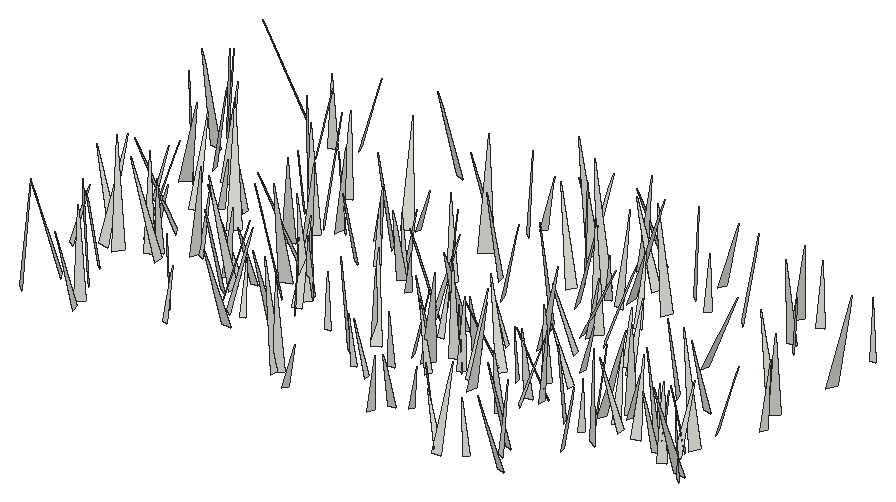
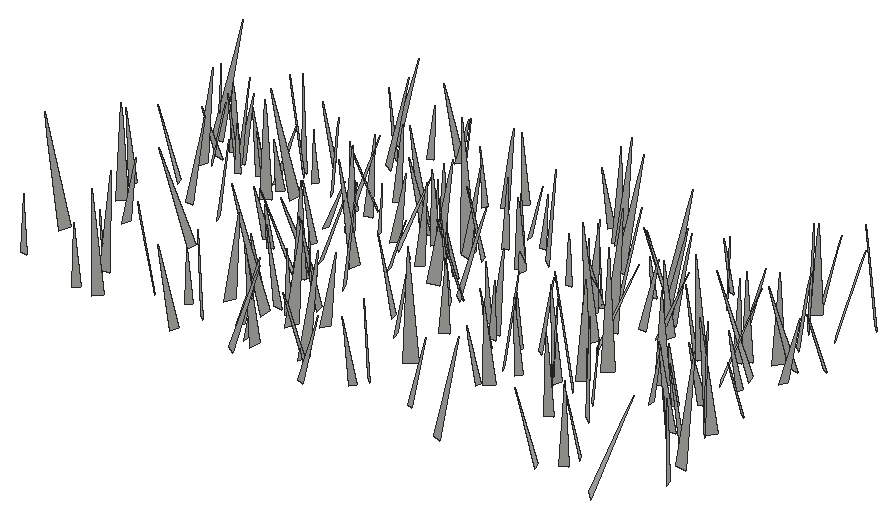
# SketchUp Ruby script. Lengths in inches.
U = 1.inch
M = Sketchup.active_model
def pt(a) = Geom::Point3d.new(a.map { |v| v * U })
def face(e, loops, mat)
  f = e.add_face(loops[0].map { |a| pt(a) })
  loops[1..].each { |l| e.add_face(l.map { |a| pt(a) }).erase! }
  f.material = f.back_material = mat if mat
  f
end
# faces: each face lists its corners as indices into pts; further lists are holes
def faces(e, pts, list, mat = nil) = list.each { |f| face(e, (f[0].is_a?(Array) ? f : [f]).map { |l| l.map { |i| pts[i] } }, mat) }
# xy, xz, yz: faces in a plane at the given z, y or x. An outline is a flat list of corners, or four numbers for a rectangle; further outlines are holes
def ring(l) = l.size == 4 ? [[l[0], l[1]], [l[2], l[1]], [l[2], l[3]], [l[0], l[3]]] : l.each_slice(2).to_a
def flat(e, list, mat, &to3) = list.each { |f| face(e, (f[0].is_a?(Array) ? f : [f]).map { |l| ring(l).map { |u, v| to3.(u, v) } }, mat) }
def xy(e, z, list, mat = nil) = flat(e, list, mat) { |x, y| [x, y, z] }
def xz(e, y, list, mat = nil) = flat(e, list, mat) { |x, z| [x, y, z] }
def yz(e, x, list, mat = nil) = flat(e, list, mat) { |y, z| [x, y, z] }
def lines(e, pts, list) = list.each { |a, b| e.add_line(pt(pts[a]), pt(pts[b])) }
# prism: a flat outline (further loops are holes) pulled along v
def prism(e, loops, v, mat = nil)
  f = face(e, loops, mat); d = Geom::Vector3d.new(v.map { |x| x * U })
  f.pushpull(f.normal.samedirection?(d) ? d.length : -d.length)
end
def box(e, o, s, mat = nil) = prism(e, [[o, [o[0] + s[0], o[1], o[2]], [o[0] + s[0], o[1] + s[1], o[2]], [o[0], o[1] + s[1], o[2]]]], [0, 0, s[2]], mat)
def at(x, y, z, deg = 0) = Geom::Transformation.translation(pt([x, y, z])) * Geom::Transformation.rotation(ORIGIN, Z_AXIS, deg.degrees)
def axes(o, x, y, z) = Geom::Transformation.new([*x, 0, *y, 0, *z, 0, *pt(o).to_a, 1])
def part(name) = M.definitions.add(name)
# library, detail: a bought-in or finely detailed component or shape, given as its bounding box
def library(name, o, s) = part(name).tap { |d| box(d.entities, o, s) }
def detail(e, o, s) = box(e.add_group.entities, o, s)
def put(e, d, t, mat = nil) = e.add_instance(d, t).tap { |i| i.material = mat if mat }
def group(e, t, mat = nil) = e.add_group.tap { |g| g.transformation = t; g.material = mat if mat }.entities
root = M.entities
c1 = part("fur_instance\#9")
p = [[0.8125,0,1.79],[0.67,-0.02,1.48],[0,-0.11,0],[0,0.11,0]]
faces(c1.entities,p,[[0,1,2,3]])
put(root,c1,axes([530.66,307.35,-21.66],[-1.81224,-5.34948,0.90018],[-5.42401,1.80193,-0.21131],[0.08596,0.92064,5.64415]))
put(root,c1,axes([467.42,306.52,-21.66],[-4.87581,-1.54153,0.97742],[-1.54685,4.96967,0.12147],[0.96896,0.17664,5.11224]))
put(root,c1,axes([498.44,307.21,-21.66],[3.31097,-1.72543,0.32906],[-1.73993,-3.31791,0.10944],[-0.24091,0.24944,3.73197]))
put(root,c1,axes([522.26,306.2,-21.66],[-3.36159,2.04077,0.19725],[2.04893,3.35754,0.1809],[0.07444,-0.25709,3.9284]))
put(root,c1,axes([459.37,306.45,-21.66],[4.78863,4.89843,2.46119],[5.13986,-5.14824,0.24599],[-1.90629,-1.57608,6.84581]))
put(root,c1,axes([522.34,305.76,-21.66],[-0.07417,5.83715,1.21265],[5.95855,0.11247,-0.17697],[0.19614,-1.2097,5.83493]))
put(root,c1,axes([525.3125,307.57,-21.66],[-2.21806,2.84038,1.31516],[3.07662,2.27502,0.2754],[0.57601,-1.21396,3.59328]))
put(root,c1,axes([509.79,309.11,-21.66],[3.72524,-2.31212,0.81738],[-2.32656,-3.80205,-0.15146],[-0.77532,0.29988,4.38182]))
put(root,c1,axes([466.73,308.3125,-21.66],[3.45962,-4.50001,2.91683],[-5.02174,-3.93643,-0.1168],[-1.88153,2.2319,5.67498]))
put(root,c1,axes([495.38,309.34,-21.66],[-7.11208,1.53537,2.26223],[1.65379,7.4363,0.15223],[2.17716,-0.6331,7.27433]))
put(root,c1,axes([495.52,309.58,-21.66],[3.10657,-5.20372,2.6425],[-5.63717,-3.45056,-0.16782],[-1.51121,2.17421,6.05816]))
put(root,c1,axes([511.11,311.35,-21.66],[1.53045,-4.60076,0.23907],[-4.60681,-1.52625,0.11946],[0.03806,0.26453,4.84716]))
put(root,c1,axes([518.17,310.44,-21.66],[-3.06281,-3.15709,1.43812],[-3.29391,3.24851,0.11628],[1.08883,0.94666,4.3971]))
put(root,c1,axes([528.46,310.15,-21.66],[-2.24155,-3.80564,2.54295],[-4.42537,2.52493,-0.12217],[1.16862,2.26183,4.41503]))
put(root,c1,axes([461.24,311.66,-21.66],[-5.49942,-3.45806,0.94275],[-3.51329,5.5426,-0.16378],[0.70973,0.64178,6.49422]))
put(root,c1,axes([477.7,310.56,-21.66],[1.06055,3.50039,1.15885],[3.68372,-1.05849,-0.17402],[-0.16095,-1.16074,3.65339]))
put(root,c1,axes([527.93,312.2,-21.66],[-2.71876,-5.31687,1.33657],[-5.469,2.73415,-0.24823],[0.3815,1.3048,5.9665]))
put(root,c1,axes([464.92,312.15,-21.66],[4.55418,4.59674,3.34406],[5.23121,-5.06575,-0.16086],[-2.22422,-2.50228,6.46875]))
put(root,c1,axes([513.14,312.56,-21.66],[3.09975,-1.98369,0.33098],[-1.98147,-3.11644,-0.1208],[-0.34401,0.07615,3.67817]))
put(root,c1,axes([483.9,314.35,-21.66],[0.0355,-6.28923,0.69696],[-6.32457,-0.05728,-0.19472],[-0.19984,0.69551,6.28631]))
put(root,c1,axes([491.09,314.8,-21.66],[-1.0754,-7.3325,1.08617],[-7.40599,1.10888,0.15329],[0.31086,1.05196,7.40935]))
put(root,c1,axes([475.96,313.58,-21.66],[3.3067,2.95122,2.18217],[3.23124,-3.73382,0.15332],[-1.74087,-1.32466,4.4295]))
put(root,c1,axes([504.39,315.08,-21.66],[-3.7389,-0.44853,0.79303],[-0.43438,3.82202,0.11371],[0.80087,-0.02096,3.764]))
put(root,c1,axes([463.32,316.11,-21.66],[-2.97615,-4.05495,1.48787],[-4.26463,3.04523,-0.23114],[0.68511,1.34083,5.02461]))
put(root,c1,axes([501.67,316.05,-21.66],[0.6335,-3.36408,1.34348],[-3.58683,-0.77327,-0.24494],[-0.50657,1.2682,3.41444]))
put(root,c1,axes([533.28,315.68,-21.66],[4.00682,1.30969,1.18737],[1.29487,-4.17692,0.23764],[-1.20352,-0.13365,4.20874]))
put(root,c1,axes([547.74,319.59,-21.66],[-0.40558,-7.48594,0.6627],[-7.51279,0.42075,0.15485],[0.19107,0.65318,7.49532]))
put(root,c1,axes([521.9,318.14,-21.66],[2.34766,-4.1804,1.05082],[-4.25289,-2.44131,-0.21062],[-0.70205,0.80976,4.78987]))
put(root,c1,axes([505.07,318.8125,-21.66],[1.42662,-4.11071,0.89066],[-4.20545,-1.41051,0.22612],[-0.07357,0.91596,4.34535]))
put(root,c1,axes([484.17,317.05,-21.66],[-1.12302,3.48075,0.37457],[3.50037,1.10997,0.18007],[-0.0574,-0.41163,3.65299]))
put(root,c1,axes([498.94,318.61,-21.66],[3.12486,4.78234,3.10342],[5.39282,-3.6275,0.15986],[-1.8492,-2.49745,5.71052]))
put(root,c1,axes([482,317.03,-21.66],[3.27247,4.57721,0.86039],[4.6176,-3.3258,0.13012],[-0.60735,-0.62316,5.62521]))
put(root,c1,axes([548.35,318.53,-21.66],[-3.07714,-3.38347,1.94932],[-3.73457,3.27489,-0.21099],[1.14047,1.59489,4.5686]))
put(root,c1,axes([535.08,319.03,-21.66],[-2.81459,-5.30869,2.75415],[-5.79641,3.17103,0.18862],[1.47279,2.33491,6.00571]))
put(root,c1,axes([457.4375,318.29,-21.66],[2.29816,3.3477,0.63042],[3.39972,-2.30202,-0.16916],[-0.21536,-0.61617,4.05709]))
put(root,c1,axes([478.39,320.55,-21.66],[-3.05463,-4.97038,1.37571],[-5.09206,3.16016,0.11108],[0.81742,1.11209,5.83293]))
put(root,c1,axes([479.4375,319.34,-21.66],[5.1332,2.66859,0.80867],[2.72409,-5.16107,-0.26035],[-0.59552,-0.60587,5.77956]))
put(root,c1,axes([534.64,319.73,-21.66],[5.13574,3.88277,2.0176],[4.11622,-5.34233,-0.19668],[-1.48436,-1.3806,6.4353]))
put(root,c1,axes([515.94,320.37,-21.66],[6.14943,-1.42717,1.61929],[-1.52874,-6.3314,0.22535],[-1.52376,0.59247,6.30885]))
put(root,c1,axes([507.93,322.17,-21.66],[6.18232,-5.30847,0.7026],[-5.32058,-6.21081,-0.10875],[-0.60412,0.37485,8.14795]))
put(root,c1,axes([532.21,320.52,-21.66],[-2.65217,1.9255,1.58872],[2.09556,2.97695,-0.10973],[1.35655,-0.83418,3.2756]))
put(root,c1,axes([509.6,320.11,-21.66],[-4.39525,1.44739,0.73649],[1.42922,4.45652,-0.22883],[0.77116,-0.01,4.62177]))
put(root,c1,axes([529.07,321.37,-21.66],[4.09073,2.15745,2.5023],[2.51133,-4.61824,-0.12369],[-2.14694,-1.2913,4.62314]))
put(root,c1,axes([544.28,320.54,-21.66],[-3.13208,3.88614,1.48189],[4.03166,3.29255,-0.11327],[1.02167,-1.07935,4.98991]))
put(root,c1,axes([542.07,322.125,-21.66],[0.17037,-4.40384,1.04145],[-4.5148,-0.2364,-0.26107],[-0.30825,1.02847,4.3994]))
put(root,c1,axes([493.76,321.06,-21.66],[-0.42673,3.51272,1.26133],[3.73148,0.37463,0.21911],[-0.0791,-1.27778,3.53176]))
put(root,c1,axes([467.84,321.62,-21.66],[-6.68615,-0.01766,0.93467],[0.01232,6.74773,0.2156],[0.93476,-0.21523,6.6827]))
put(root,c1,axes([462.76,320.43,-21.66],[-5.4488,4.52209,1.619],[4.59694,5.6194,-0.22458],[1.39234,-0.85616,7.07731]))
put(root,c1,axes([479.05,321.7,-21.66],[-7.32255,-0.11088,1.35528],[-0.08815,7.44603,0.13288],[1.35695,-0.11461,7.32218]))
put(root,c1,axes([488.25,321.68,-21.66],[-3.74017,-2.83655,2.38458],[-3.12746,4.23356,0.13062],[1.98777,1.32365,4.69232]))
put(root,c1,axes([499.97,321.9375,-21.66],[-4.58199,0.67037,2.42399],[0.81188,5.16228,0.10702],[2.38033,-0.47034,4.62953]))
put(root,c1,axes([522.46,322.8125,-21.66],[1.7038,-4.78318,1.39426],[-4.94528,-1.80274,-0.14134],[-0.60574,1.26373,5.0756]))
put(root,c1,axes([543.2,321.7,-21.66],[3.76786,2.01641,1.4087],[2.07515,-3.9894,0.15999],[-1.32064,-0.51569,4.27049]))
put(root,c1,axes([522.62,320.92,-21.66],[3.07177,3.42083,0.35758],[3.42072,-3.08846,0.16062],[-0.35863,-0.15826,4.59478]))
put(root,c1,axes([507.41,323.25,-21.66],[-0.73911,-5.79285,1.55471],[-5.99778,0.70592,-0.22109],[-0.03032,1.57006,5.83563]))
put(root,c1,axes([466.78,323.17,-21.66],[0.54293,-5.17192,1.62827],[-5.42158,-0.49338,0.24063],[0.08095,1.64396,5.19477]))
put(root,c1,axes([460.59,320.35,-21.66],[0.90222,6.95991,0.72818],[6.98982,-0.93156,0.24337],[-0.33621,-0.69025,7.01392]))
put(root,c1,axes([524.17,324.27,-21.66],[-3.22391,-4.50813,0.36238],[-4.51102,3.23719,0.13952],[0.32445,0.21334,5.54053]))
put(root,c1,axes([505.49,322.5,-21.66],[4.51759,1.55237,1.02195],[1.60919,-4.61101,-0.10928],[-0.92991,-0.4377,4.77562]))
put(root,c1,axes([480.32,324.07,-21.66],[-0.08561,-4.51883,0.61864],[-4.55746,0.06047,-0.18896],[-0.17898,0.62161,4.51569]))
put(root,c1,axes([466.05,322.18,-21.66],[-2.20554,5.93145,2.00046],[6.2413,2.24627,0.22087],[0.47966,-1.95462,6.32437]))
put(root,c1,axes([500.67,321.5625,-21.66],[-3.10471,5.12305,0.88051],[5.18598,3.12286,0.11631],[0.35573,-0.81381,5.98927]))
put(root,c1,axes([484.55,323.83,-21.66],[-5.73221,-5.07274,1.73381],[-5.23258,5.8463,-0.19467],[1.1657,1.29813,7.652]))
put(root,c1,axes([512.32,322.89,-21.66],[2.78644,2.89477,1.9564],[3.12581,-3.18339,0.25829],[-1.56092,-1.20736,4.00964]))
put(root,c1,axes([541.58,323.13,-21.66],[-6.14594,-1.15799,1.95321],[-1.28361,6.42082,-0.2323],[1.87305,0.60056,6.24977]))
put(root,c1,axes([514.49,321.92,-21.66],[0.1573,5.82785,1.1486],[5.93788,-0.12389,-0.18455],[0.15705,-1.15268,5.82705]))
put(root,c1,axes([512.07,323.25,-21.66],[-2.98009,3.50221,2.17702],[3.82104,3.35523,-0.16707],[1.55067,-1.53712,4.59549]))
put(root,c1,axes([476.6,323.46,-21.66],[4.38951,-2.01268,1.547],[-2.15257,-4.58905,0.13732],[-1.34555,0.7756,4.82698]))
put(root,c1,axes([524.23,323.125,-21.66],[4.53301,0.32886,1.81446],[0.26511,-4.88148,0.22244],[-1.82486,0.10775,4.53948]))
put(root,c1,axes([535.8,323.46,-21.66],[-4.77809,0.40303,0.49366],[0.4272,4.79644,0.21897],[0.47289,-0.2608,4.79006]))
put(root,c1,axes([544.7,324.4,-21.66],[-3.48684,-2.54111,1.02639],[-2.66037,3.53733,-0.28017],[0.65812,0.83597,4.30544]))
put(root,c1,axes([459.46,323.64,-21.66],[-4.99004,2.24313,0.58277],[2.2784,5.00139,0.2583],[0.42444,-0.4756,5.46492]))
put(root,c1,axes([538.38,323.07,-21.66],[-2.22109,4.73282,1.14399],[4.81333,2.32397,-0.26934],[0.73496,-0.91711,5.22114]))
put(root,c1,axes([477.6875,324.09,-21.66],[-5.92651,0.06077,0.05927],[0.05827,5.92175,-0.24529],[0.06173,0.24468,5.92174]))
put(root,c1,axes([544.89,322.75,-21.66],[0.14678,4.73777,0.12743],[4.7339,-0.15274,0.22615],[-0.23006,-0.12022,4.73465]))
put(root,c1,axes([531.96,324.78,-21.66],[6.74375,-1.56753,0.95704],[-1.61805,-6.79399,0.27364],[-0.86892,0.48558,6.91813]))
put(root,c1,axes([470.56,325.22,-21.66],[5.91489,-2.56905,1.81184],[-2.61095,-6.16477,-0.21752],[-1.75092,0.51416,6.44505]))
put(root,c1,axes([540.88,324.26,-21.66],[-1.02276,3.4571,1.0392],[3.60758,1.01767,0.16502],[0.12981,-1.04418,3.60144]))
put(root,c1,axes([487.22,325.95,-21.66],[2.10827,-4.41232,0.88185],[-4.4927,-2.11805,0.1432],[-0.24874,0.85808,4.88803]))
put(root,c1,axes([509.66,324.89,-21.66],[-1.05184,5.80364,2.59591],[6.34975,1.09094,0.13387],[0.3189,-2.57972,5.89666]))
put(root,c1,axes([487.54,324.6,-21.66],[-5.4066,3.91291,1.98693],[4.14231,5.59139,0.26032],[1.44915,-1.38406,6.66892]))
put(root,c1,axes([487.61,322.93,-21.66],[-1.13883,5.42731,0.08742],[5.42427,1.13458,0.2244],[-0.2017,-0.13157,5.54096]))
put(root,c1,axes([482.97,326.68,-21.66],[2.46891,-7.20313,1.70316],[-7.36136,-2.57683,-0.22704],[-0.77207,1.53499,7.61111]))
put(root,c1,axes([514.81,326.84,-21.66],[-3.4454,-3.89131,0.03074],[-3.88746,3.44363,0.20759],[0.17579,-0.11462,5.19326]))
put(root,c1,axes([518.83,325.27,-21.66],[3.01328,1.01562,1.71575],[1.06477,-3.44849,0.1713],[-1.68569,-0.36275,3.17522]))
put(root,c1,axes([471.23,325.33,-21.66],[1.95636,4.4496,1.57567],[4.70552,-1.97342,-0.26957],[-0.3738,-1.55425,4.8532]))
put(root,c1,axes([487.67,325.6,-21.66],[2.36348,3.65871,1.87372],[3.9267,-2.64879,0.21906],[-1.21573,-1.4425,4.3502]))
put(root,c1,axes([534.76,326.47,-21.66],[3.71508,-1.29272,0.27873],[-1.28155,-3.72443,-0.19222],[-0.32626,-0.0905,3.92887]))
put(root,c1,axes([462.98,325.3,-21.66],[6.72571,2.73267,0.89443],[2.78268,-6.75899,-0.27437],[-0.72399,-0.59256,7.25447]))
put(root,c1,axes([534.37,324.48,-21.66],[-2.34195,3.99616,0.3444],[3.99913,2.35703,-0.15486],[0.30802,-0.21845,4.62925]))
put(root,c1,axes([545.4,325.4,-21.66],[-6.9298,2.98954,1.57704],[3.02348,7.09089,-0.15622],[1.51094,-0.47802,7.54553]))
put(root,c1,axes([521.89,326.9375,-21.66],[4.08918,-3.36848,1.98263],[-3.52303,-4.41912,-0.24183],[-1.69286,1.05996,5.29241]))
put(root,c1,axes([510.38,328.24,-21.66],[2.722,-4.21365,0.18087],[-4.20663,-2.72794,-0.24377],[-0.30292,0.01939,5.01046]))
put(root,c1,axes([465.27,328.2,-21.66],[-5.5722,-4.07145,0.43281],[-4.071,5.58734,0.1482],[0.43699,0.13539,6.89957]))
put(root,c1,axes([516.1,325.6875,-21.66],[-4.785,3.6619,0.62252],[3.69492,4.79647,0.18627],[0.38032,-0.52686,6.02254]))
put(root,c1,axes([534.39,327.08,-21.66],[-1.98157,5.41612,3.08152],[6.10168,2.34277,-0.19399],[1.26474,-2.81671,5.76397]))
put(root,c1,axes([462.39,328.2,-21.66],[3.14021,-1.95272,0.11029],[-1.95573,-3.13292,0.21476],[0.01996,0.24059,3.6916]))
put(root,c1,axes([506.39,330.7,-21.66],[2.6634,-7.09113,0.13913],[-7.08626,-2.66678,-0.26525],[-0.29724,0.03689,7.57017]))
put(root,c1,axes([524.63,328.01,-21.66],[-3.98782,0.86871,0.11292],[0.87287,3.98492,0.16912],[0.07423,-0.18933,4.07783]))
put(root,c1,axes([505.36,327.8,-21.66],[0.0321,3.78164,0.61426],[3.82721,-0.05969,0.16749],[-0.17489,-0.6122,3.77806]))
put(root,c1,axes([483.15,329.96,-21.66],[6.93717,-2.75986,2.51351],[-2.97128,-7.29338,0.19237],[-2.25967,1.11744,7.46352]))
put(root,c1,axes([481.44,331.18,-21.66],[-5.39414,-3.77764,0.22745],[-3.78403,5.38986,-0.22257],[0.05845,0.31282,6.58162]))
put(root,c1,axes([501.96,331.6,-21.66],[-3.86878,-4.9807,0.99535],[-5.05831,3.89149,-0.18804],[0.45997,0.9025,6.30392]))
put(root,c1,axes([544.89,330.22,-21.66],[4.65489,2.00226,0.76997],[2.06003,-4.68544,-0.26978],[-0.59848,-0.55448,5.06006]))
put(root,c1,axes([512.64,331.13,-21.66],[-3.89073,-0.42692,0.42553],[-0.44504,3.90915,-0.14719],[0.40654,0.19356,3.91132]))
put(root,c1,axes([523.32,331.94,-21.66],[3.83276,-0.80553,0.30542],[-0.78769,-3.84079,-0.24507],[-0.34886,-0.17786,3.90882]))
put(root,c1,axes([540.79,333.45,-21.66],[-1.08369,-5.40972,1.03151],[-5.49173,1.14023,0.21038],[0.41232,0.96864,5.51318]))
put(root,c1,axes([501.6,331.24,-21.66],[3.62165,4.35293,0.90177],[4.41878,-3.65214,-0.11732],[-0.48531,-0.76904,5.66132]))
put(root,c1,axes([477.28,334.29,-21.66],[4.02071,-6.30995,0.86141],[-6.36147,-4.02715,0.19326],[-0.29869,0.83076,7.47959]))
put(root,c1,axes([516.22,333.16,-21.66],[6.40795,-1.734,1.03011],[-1.73088,-6.48917,-0.15614],[-1.03535,0.11648,6.63658]))
put(root,c1,axes([495.57,333.9375,-21.66],[2.79472,-2.37927,0.19168],[-2.37504,-2.80125,-0.14262],[-0.23842,0.01542,3.66757]))
put(root,c1,axes([458.3,332.66,-21.66],[2.21445,2.95218,0.72503],[3.03203,-2.20951,-0.26401],[-0.21871,-0.73996,3.68096]))
put(root,c1,axes([501.79,333.32,-21.66],[5.69134,3.55142,2.30083],[3.82093,-5.97012,-0.23634],[-1.81848,-1.42926,6.70433]))
put(root,c1,axes([535.89,334.13,-21.66],[4.40996,1.53054,2.75088],[1.88618,-5.07543,-0.19988],[-2.52036,-1.1203,4.66373]))
put(root,c1,axes([548.86,334.06,-21.66],[4.44334,-1.86269,1.64457],[-2.02269,-4.66849,0.17731],[-1.44323,0.80817,4.81471]))
put(root,c1,axes([520.02,334.68,-21.66],[-4.58656,-0.99691,0.53395],[-0.9871,4.61746,0.14195],[0.55187,-0.02624,4.69151]))
put(root,c1,axes([493.13,335.72,-21.66],[2.16413,-4.87719,1.14426],[-4.95965,-2.26151,-0.2591],[-0.70577,0.93721,5.32947]))
put(root,c1,axes([470.29,332.83,-21.66],[-5.1988,6.07272,1.14347],[6.1224,5.26442,-0.12263],[0.83765,-0.78798,7.99315]))
put(root,c1,axes([486.35,335.67,-21.66],[-2.7828,-3.97435,1.2381],[-4.07565,2.90431,0.16237],[0.84701,0.91751,4.84903]))
put(root,c1,axes([465.95,335.78,-21.66],[3.13443,-2.25979,0.73802],[-2.32723,-3.16608,0.18952],[-0.4851,0.5876,3.85946]))
put(root,c1,axes([463.53,333.66,-21.66],[-2.14385,5.53708,0.23418],[5.53457,2.15208,-0.21752],[0.2875,-0.13964,5.93364]))
put(root,c1,axes([528.35,334.49,-21.66],[-1.52341,4.48001,0.30788],[4.47725,1.54034,-0.26007],[0.34571,-0.20714,4.72479]))
put(root,c1,axes([492.76,336.62,-21.66],[-0.42877,3.87256,1.55947],[4.17346,0.35848,0.25729],[-0.1042,-1.57711,3.88772]))
put(root,c1,axes([526.67,335.92,-21.66],[-1.83169,3.1238,0.57494],[3.14275,1.87858,-0.19441],[0.4602,-0.39568,3.61599]))
put(root,c1,axes([468.62,336.93,-21.66],[-3.8802,0.07929,1.10053],[0.11582,4.03064,0.11798],[1.09728,-0.14508,3.87922]))
put(root,c1,axes([488.75,336.62,-21.66],[-3.06481,2.41196,1.362],[2.48233,3.29293,-0.24563],[1.22908,-0.63618,3.89234]))
put(root,c1,axes([458.44,338.36,-21.66],[5.57249,-4.36069,0.56036],[-4.38496,-5.5781,0.19774],[-0.31889,0.50141,7.07313]))
put(root,c1,axes([547.42,337.86,-21.66],[-3.8078,3.44308,3.43375],[4.19662,4.52997,0.11149],[2.45637,-2.40193,5.13242]))
put(root,c1,axes([513.98,337.91,-21.66],[-6.04607,-3.24149,2.31572],[-3.3744,6.40425,0.15438],[2.11738,0.95032,6.85845]))
put(root,c1,axes([478.23,337.77,-21.66],[-4.52139,5.22079,2.42729],[5.56937,4.74843,0.161],[1.45961,-1.94607,6.90462]))
put(root,c1,axes([459.07,339,-21.66],[-4.9247,-5.05159,2.9073],[-5.39927,5.38751,0.21521],[2.19519,1.91829,7.05159]))
put(root,c1,axes([518.82,338.69,-21.66],[4.01363,-0.60213,1.19124],[-0.70216,-4.16285,0.26162],[-1.13516,0.446,4.0501]))
put(root,c1,axes([491.41,338.9,-21.66],[3.83893,-0.81047,1.08867],[-0.8917,-3.9684,0.19003],[-1.0232,0.41758,3.91895]))
put(root,c1,axes([518.03,338.52,-21.66],[5.44846,0.74036,0.07595],[0.73692,-5.44519,0.21553],[-0.10422,0.20337,5.4943]))
put(root,c1,axes([521.3,338.55,-21.66],[4.74716,3.3592,0.52437],[3.38285,-4.75689,-0.1518],[-0.33985,-0.42721,5.81349]))
put(root,c1,axes([480.22,340.1,-21.66],[5.9168,-1.45412,1.7202],[-1.44139,-6.15974,-0.24915],[-1.73089,0.15879,6.08776]))
put(root,c1,axes([498.02,339.09,-21.66],[2.13883,-4.28297,3.06723],[-5.00629,-2.68295,-0.2554],[-1.63976,2.60467,4.7805]))
put(root,c1,axes([505.16,339.63,-21.66],[5.01565,1.80166,1.23073],[1.89818,-5.12441,-0.23415],[-1.07592,-0.64182,5.32428]))
put(root,c1,axes([480.64,340.59,-21.66],[-3.25997,-4.21096,1.97124],[-4.4396,3.53441,0.20814],[1.38129,1.42168,5.3213]))
put(root,c1,axes([484.92,341.45,-21.66],[3.8804,-2.67072,0.47699],[-2.66948,-3.90717,-0.15997],[-0.48385,0.13783,4.70793]))
put(root,c1,axes([487.4,341.15,-21.66],[-5.57513,-2.9786,1.92177],[-3.03694,5.86084,0.2736],[1.82819,0.65252,6.315]))
put(root,c1,axes([519.27,339.77,-21.66],[-5.69,4.35692,2.08043],[4.49689,5.95288,-0.16772],[1.75752,-1.1258,7.16454]))
put(root,c1,axes([477.97,340.07,-21.66],[5.88152,4.86813,2.28116],[5.13014,-6.09312,-0.22398],[-1.60749,-1.63397,7.63157]))
put(root,c1,axes([473.96,341.39,-21.66],[-3.08736,-2.6391,1.38175],[-2.74426,3.29386,0.15946],[1.15895,0.7691,4.05847]))
put(root,c1,axes([534.06,341.42,-21.66],[6.32443,-0.86949,0.03215],[-0.87008,-6.31952,0.24926],[0.00213,0.25131,6.37905]))
put(root,c1,axes([474.44,341.64,-21.66],[2.40837,2.51325,1.53163],[2.71206,-2.66382,0.10655],[-1.14326,-1.0248,3.47927]))
put(root,c1,axes([462.55,340.93,-21.66],[-0.45657,6.34549,1.8425],[6.59681,0.54314,-0.23589],[0.37708,-1.81886,6.35752]))
put(root,c1,axes([543.77,341.6,-21.66],[-4.87029,1.64927,0.93909],[1.65484,4.95663,-0.12272],[0.92923,-0.18296,5.1405]))
put(root,c1,axes([502.15,343.06,-21.66],[-5.31437,-1.63311,1.48269],[-1.72892,5.48589,-0.1545],[1.36976,0.58821,5.55749]))
put(root,c1,axes([459.34,342.84,-21.66],[5.12051,1.66894,1.66295],[1.70709,-5.37015,0.13306],[-1.62376,-0.38277,5.38398]))
put(root,c1,axes([513.03,343.8,-21.66],[5.83146,1.27805,1.15338],[1.33487,-5.92923,-0.17895],[-1.08712,-0.42484,5.96719]))
put(root,c1,axes([472.03,344.78,-21.66],[3.78368,4.97369,3.03573],[5.56614,-4.15585,-0.12867],[-1.72376,-2.50217,6.24798]))
put(root,c1,axes([522,343.89,-21.66],[-1.31854,4.49628,0.43937],[4.51767,1.31381,0.11263],[0.01505,-0.45333,4.68427]))
put(root,c1,axes([456.17,346.95,-21.66],[-0.95753,-7.17721,1.84222],[-7.39469,1.0444,0.22542],[0.47406,1.79439,7.23729]))
put(root,c1,axes([487.26,346.18,-21.66],[3.61055,-0.61097,0.20103],[-0.59508,-3.6081,-0.27795],[-0.24409,-0.24103,3.65131]))
put(root,c1,axes([515.02,347.13,-21.66],[2.03296,-3.43324,0.36978],[-3.45285,-2.01606,0.26469],[0.04074,0.45292,3.9812]))
put(root,c1,axes([548.43,347.26,-21.66],[6.87118,-2.4682,1.14103],[-2.53265,-6.93781,0.24398],[-0.98977,0.61792,7.29696]))
put(root,c1,axes([486.15,345.46,-21.66],[-3.98192,5.65644,1.02142],[5.69703,4.04883,-0.21229],[0.76316,-0.7113,6.91418]))
put(root,c1,axes([476.07,346.9,-21.66],[-2.39493,4.93051,2.15105],[5.27679,2.61079,-0.10925],[1.04521,-1.88321,5.4803]))
put(root,c1,axes([496.72,347,-21.66],[4.92232,-5.34816,3.43981],[-5.97476,-5.37881,0.1869],[-2.17654,2.67018,7.26616]))
put(root,c1,axes([517.0625,346.49,-21.66],[1.06492,5.99669,1.55027],[6.17359,-1.15473,0.22589],[-0.50038,-1.48458,6.08632]))
put(root,c1,axes([509.93,346.51,-21.66],[-5.57386,3.34507,0.61319],[3.34749,5.6042,-0.14346],[0.5998,-0.19191,6.49898]))
put(root,c1,axes([517.41,348.4375,-21.66],[8.28106,0.30024,0.90595],[0.31898,-8.32832,-0.15571],[-0.89952,-0.18935,8.28504]))
put(root,c1,axes([510.06,348.9,-21.66],[4.77754,4.17311,2.72058],[4.61145,-5.13068,-0.22808],[-1.8844,-1.97551,6.33938]))
put(root,c1,axes([522.66,348.57,-21.66],[-6.31107,2.62453,1.38258],[2.63294,6.45317,-0.23139],[1.36651,-0.31261,6.83112]))
put(root,c1,axes([513.21,348.77,-21.66],[-7.4138,3.10521,1.79195],[3.13289,7.61249,-0.22981],[1.74312,-0.47482,8.03455]))
put(root,c1,axes([456.03,349.375,-21.66],[3.99026,4.07334,2.14881],[4.32029,-4.29562,0.12027],[-1.59518,-1.44473,5.70086]))
put(root,c1,axes([455.0625,350.76,-21.66],[-4.85936,-1.80324,2.4582],[-1.94231,5.39639,0.11902],[2.34986,0.73149,5.18178]))
put(root,c1,axes([539.9375,350.73,-21.66],[-2.43911,-2.15453,1.73505],[-2.51562,2.68975,-0.19638],[1.15067,1.31336,3.24849]))
put(root,c1,axes([538.45,352.35,-21.66],[0.4786,-6.17329,1.68247],[-6.39725,-0.42884,0.2463],[0.12453,1.69584,6.18692]))
put(root,c1,axes([525.85,352.23,-21.66],[-2.23187,2.81976,1.51549],[3.01775,2.4697,-0.15093],[1.06816,-1.08561,3.59298]))
put(root,c1,axes([466.8,352.57,-21.66],[4.26525,2.34746,1.0733],[2.44325,-4.34035,-0.2164],[-0.83252,-0.71113,4.86375]))
put(root,c1,axes([518.05,352.34,-21.66],[-5.4054,2.23783,0.44972],[2.26041,5.40869,0.2551],[0.31726,-0.40826,5.84475]))
put(root,c1,axes([530.82,352.57,-21.66],[-3.67972,-3.6806,3.42599],[-4.33109,4.47676,0.15761],[2.55458,2.28831,5.20214]))
put(root,c1,axes([498.01,353.29,-21.66],[3.30572,4.13092,2.03155],[4.38871,-3.58299,0.14433],[-1.38957,-1.489,5.28881]))
put(root,c1,axes([490.24,355.27,-21.66],[-1.40933,-4.17013,0.64925],[-4.20295,1.44894,0.18319],[0.38311,0.55526,4.39803]))
put(root,c1,axes([522.62,353.8,-21.66],[3.82157,4.19761,2.25189],[4.45533,-4.17126,0.21447],[-1.68552,-1.50865,5.67259]))
put(root,c1,axes([507.04,354.16,-21.66],[-7.37907,1.498,2.27835],[1.63074,7.6926,0.22378],[2.18531,-0.6822,7.52626]))
put(root,c1,axes([467.23,355.2,-21.66],[1.77747,-4.94769,1.74658],[-5.22789,-1.82695,0.145],[-0.44649,1.69476,5.25529]))
put(root,c1,axes([515.35,354.71,-21.66],[-3.60239,-0.15597,0.87969],[-0.19043,3.7046,-0.12301],[0.87288,0.16452,3.60367]))
put(root,c1,axes([548.5,354.99,-21.66],[-0.06677,3.94377,1.582],[4.24655,0.00562,0.16522],[-0.15123,-1.5834,3.94087]))
put(root,c1,axes([498.66,355.48,-21.66],[3.79566,-1.87078,0.73995],[-1.92959,-3.83243,0.2087],[-0.56925,0.51676,4.2265]))
put(root,c1,axes([513.58,355.21,-21.66],[6.28963,-0.96384,2.1084],[-1.07131,-6.61487,0.17192],[-2.05588,0.49827,6.36073]))
put(root,c1,axes([506.45,354.75,-21.66],[2.03381,4.83721,0.83738],[4.90479,-2.04045,-0.1258],[-0.20703,-0.82108,5.24587]))
put(root,c1,axes([535.49,357.35,-21.66],[5.23742,-3.794,0.7561],[-3.79638,-5.28528,-0.22367],[-0.74406,0.26094,6.46336]))
put(root,c1,axes([515.09,357.76,-21.66],[-2.82637,-5.01502,0.69558],[-5.06125,2.81969,-0.23605],[0.13409,0.7222,5.75179]))
put(root,c1,axes([460.44,358.77,-21.66],[-5.16383,-5.19186,0.43743],[-5.2089,5.15828,-0.26709],[0.11856,0.49863,7.31773]))
put(root,c1,axes([469.76,357.15,-21.66],[4.69401,2.26049,0.88712],[2.32694,-4.7392,-0.23643],[-0.69438,-0.60059,5.20458]))
put(root,c1,axes([504,358.67,-21.66],[-1.28236,-4.10189,0.60594],[-4.14572,1.27987,-0.10961],[0.07509,0.61118,4.29626]))
put(root,c1,axes([523.41,358.03,-21.66],[4.86131,-2.02952,0.59697],[-2.06386,-4.87843,0.22145],[-0.46454,0.43544,5.26329]))
put(root,c1,axes([538.64,357.39,-21.66],[-2.37433,3.47563,1.70417],[3.72029,2.6012,-0.12184],[1.06942,-1.33243,4.20745]))
put(root,c1,axes([483.01,359.2,-21.66],[-2.27159,-6.08211,1.19958],[-6.16809,2.34544,0.21162],[0.62109,1.04786,6.48903]))
